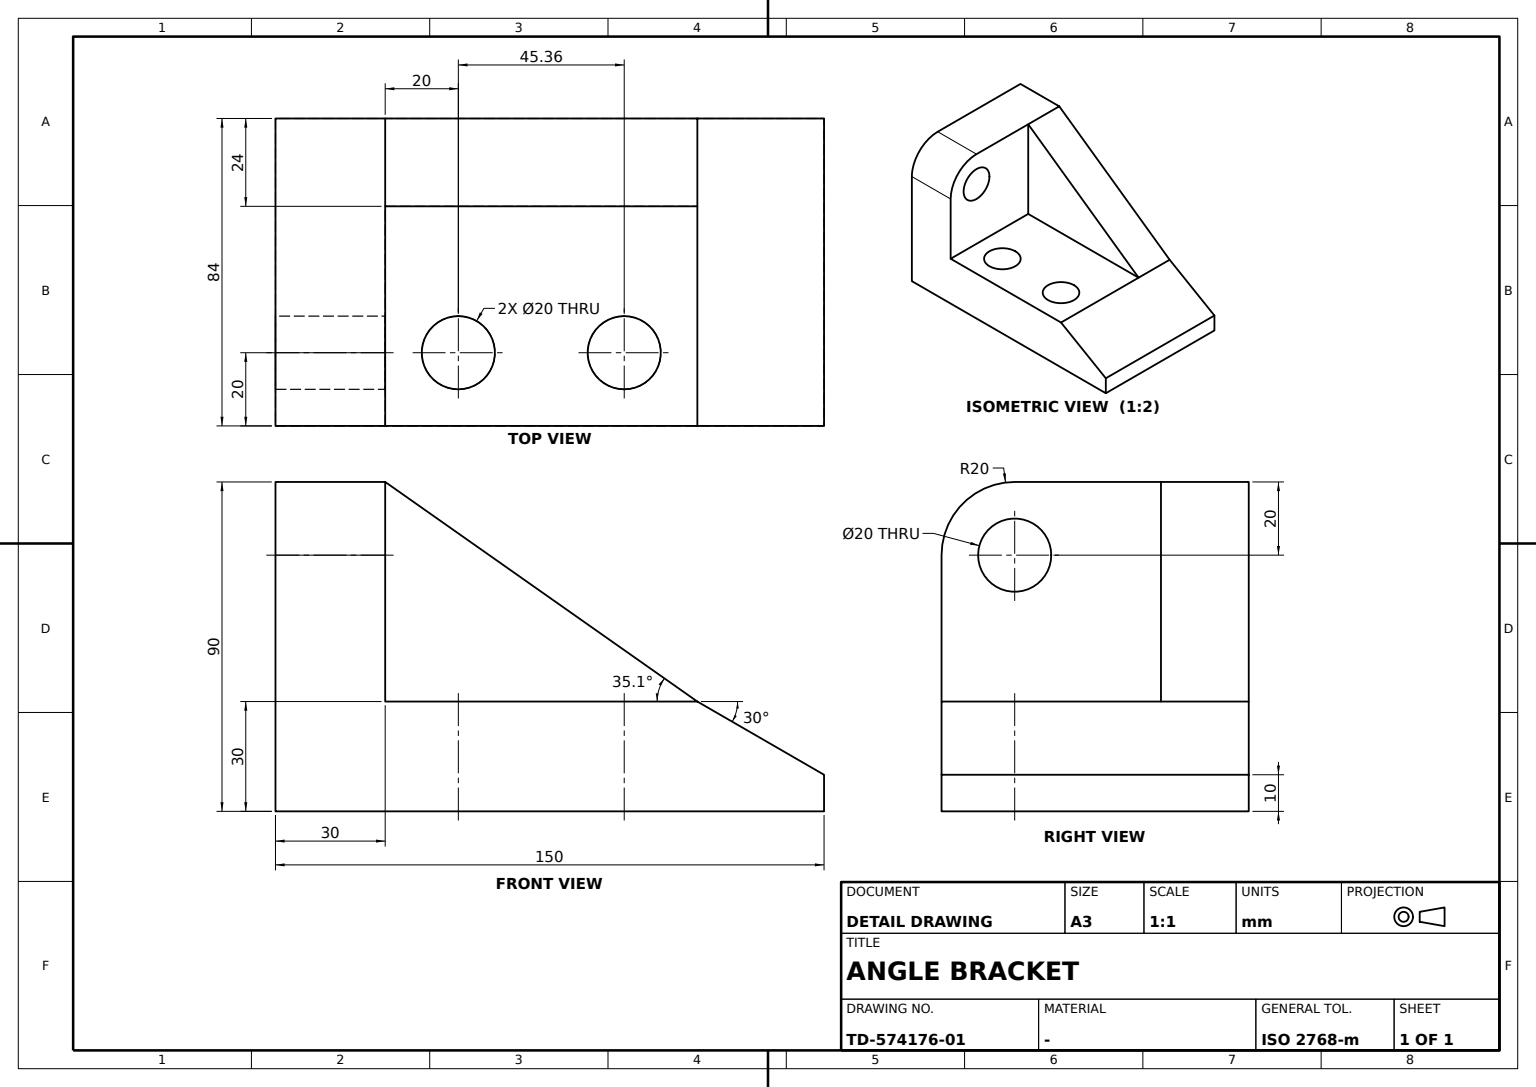
ISO-10303-21;
HEADER;
FILE_DESCRIPTION((''),'2;1');
FILE_NAME('','',(''),(''),'','','');
FILE_SCHEMA(('AUTOMOTIVE_DESIGN'));
ENDSEC;
DATA;
#1=APPLICATION_CONTEXT('');
#2=PRODUCT_CONTEXT('',#1,'mechanical');
#3=PRODUCT('','','',(#2));
#4=PRODUCT_DEFINITION_FORMATION('','',#3);
#5=PRODUCT_DEFINITION_CONTEXT('',#1,'design');
#6=PRODUCT_DEFINITION('','',#4,#5);
#7=PRODUCT_DEFINITION_SHAPE('','',#6);
#8=(LENGTH_UNIT()NAMED_UNIT(*)SI_UNIT(.MILLI.,.METRE.));
#9=(NAMED_UNIT(*)PLANE_ANGLE_UNIT()SI_UNIT($,.RADIAN.));
#10=(NAMED_UNIT(*)SI_UNIT($,.STERADIAN.)SOLID_ANGLE_UNIT());
#11=UNCERTAINTY_MEASURE_WITH_UNIT(LENGTH_MEASURE(1.E-05),#8,'distance_accuracy_value','');
#12=(GEOMETRIC_REPRESENTATION_CONTEXT(3)GLOBAL_UNCERTAINTY_ASSIGNED_CONTEXT((#11))GLOBAL_UNIT_ASSIGNED_CONTEXT((#8,#9,#10))REPRESENTATION_CONTEXT('',''));
#13=CARTESIAN_POINT('',(42.,150.,10.));
#14=VERTEX_POINT('',#13);
#15=CARTESIAN_POINT('',(-42.,150.,10.));
#16=VERTEX_POINT('',#15);
#17=CARTESIAN_POINT('',(0.,150.,10.));
#18=DIRECTION('',(-1.,0.,0.));
#19=VECTOR('',#18,1000.);
#20=LINE('',#17,#19);
#21=EDGE_CURVE('',#14,#16,#20,.T.);
#22=ORIENTED_EDGE('',*,*,#21,.F.);
#23=CARTESIAN_POINT('',(42.,150.,0.));
#24=VERTEX_POINT('',#23);
#25=CARTESIAN_POINT('',(42.,150.,5.));
#26=DIRECTION('',(0.,0.,1.));
#27=VECTOR('',#26,1000.);
#28=LINE('',#25,#27);
#29=EDGE_CURVE('',#24,#14,#28,.T.);
#30=ORIENTED_EDGE('',*,*,#29,.F.);
#31=CARTESIAN_POINT('',(-42.,150.,0.));
#32=VERTEX_POINT('',#31);
#33=CARTESIAN_POINT('',(0.,150.,0.));
#34=DIRECTION('',(1.,0.,0.));
#35=VECTOR('',#34,1000.);
#36=LINE('',#33,#35);
#37=EDGE_CURVE('',#32,#24,#36,.T.);
#38=ORIENTED_EDGE('',*,*,#37,.F.);
#39=CARTESIAN_POINT('',(-42.,150.,5.));
#40=LINE('',#39,#27);
#41=EDGE_CURVE('',#32,#16,#40,.T.);
#42=ORIENTED_EDGE('',*,*,#41,.T.);
#43=EDGE_LOOP('',(#22,#30,#38,#42));
#44=FACE_OUTER_BOUND('',#43,.T.);
#45=DIRECTION('',(0.,1.,0.));
#46=AXIS2_PLACEMENT_3D('',#33,#45,#26);
#47=PLANE('',#46);
#48=ADVANCED_FACE('',(#44),#47,.T.);
#49=CARTESIAN_POINT('',(-18.,30.,30.));
#50=VERTEX_POINT('',#49);
#51=CARTESIAN_POINT('',(42.,30.,30.));
#52=VERTEX_POINT('',#51);
#53=CARTESIAN_POINT('',(12.,30.,30.));
#54=LINE('',#53,#35);
#55=EDGE_CURVE('',#50,#52,#54,.T.);
#56=ORIENTED_EDGE('',*,*,#55,.F.);
#57=CARTESIAN_POINT('',(-18.,30.,90.));
#58=VERTEX_POINT('',#57);
#59=CARTESIAN_POINT('',(-18.,30.,60.));
#60=DIRECTION('',(0.,0.,-1.));
#61=VECTOR('',#60,1000.);
#62=LINE('',#59,#61);
#63=EDGE_CURVE('',#58,#50,#62,.T.);
#64=ORIENTED_EDGE('',*,*,#63,.F.);
#65=CARTESIAN_POINT('',(22.,30.,90.));
#66=VERTEX_POINT('',#65);
#67=CARTESIAN_POINT('',(2.,30.,90.));
#68=LINE('',#67,#35);
#69=EDGE_CURVE('',#58,#66,#68,.T.);
#70=ORIENTED_EDGE('',*,*,#69,.T.);
#71=CARTESIAN_POINT('',(42.,30.,70.));
#72=VERTEX_POINT('',#71);
#73=CARTESIAN_POINT('',(22.,30.,70.));
#74=DIRECTION('',(0.,-1.,0.));
#75=AXIS2_PLACEMENT_3D('',#73,#74,#60);
#76=CIRCLE('',#75,20.);
#77=EDGE_CURVE('',#72,#66,#76,.T.);
#78=ORIENTED_EDGE('',*,*,#77,.F.);
#79=CARTESIAN_POINT('',(42.,30.,50.));
#80=LINE('',#79,#27);
#81=EDGE_CURVE('',#52,#72,#80,.T.);
#82=ORIENTED_EDGE('',*,*,#81,.F.);
#83=EDGE_LOOP('',(#56,#64,#70,#78,#82));
#84=FACE_OUTER_BOUND('',#83,.T.);
#85=CARTESIAN_POINT('',(12.,30.,70.));
#86=VERTEX_POINT('',#85);
#87=CARTESIAN_POINT('',(32.,30.,70.));
#88=VERTEX_POINT('',#87);
#89=AXIS2_PLACEMENT_3D('',#73,#45,#18);
#90=CIRCLE('',#89,10.);
#91=EDGE_CURVE('',#86,#88,#90,.T.);
#92=ORIENTED_EDGE('',*,*,#91,.F.);
#93=EDGE_CURVE('',#88,#86,#90,.T.);
#94=ORIENTED_EDGE('',*,*,#93,.F.);
#95=EDGE_LOOP('',(#92,#94));
#96=FACE_BOUND('',#95,.T.);
#97=CARTESIAN_POINT('',(0.,30.,90.));
#98=AXIS2_PLACEMENT_3D('',#97,#74,#60);
#99=PLANE('',#98);
#100=ADVANCED_FACE('',(#84,#96),#99,.F.);
#101=ORIENTED_EDGE('',*,*,#41,.F.);
#102=CARTESIAN_POINT('',(-42.,0.,0.));
#103=VERTEX_POINT('',#102);
#104=CARTESIAN_POINT('',(-42.,75.,0.));
#105=VECTOR('',#45,1000.);
#106=LINE('',#104,#105);
#107=EDGE_CURVE('',#103,#32,#106,.T.);
#108=ORIENTED_EDGE('',*,*,#107,.F.);
#109=CARTESIAN_POINT('',(-42.,0.,90.));
#110=VERTEX_POINT('',#109);
#111=CARTESIAN_POINT('',(-42.,0.,45.));
#112=LINE('',#111,#61);
#113=EDGE_CURVE('',#110,#103,#112,.T.);
#114=ORIENTED_EDGE('',*,*,#113,.F.);
#115=CARTESIAN_POINT('',(-42.,30.,90.));
#116=VERTEX_POINT('',#115);
#117=CARTESIAN_POINT('',(-42.,15.,90.));
#118=VECTOR('',#74,1000.);
#119=LINE('',#117,#118);
#120=EDGE_CURVE('',#116,#110,#119,.T.);
#121=ORIENTED_EDGE('',*,*,#120,.F.);
#122=CARTESIAN_POINT('',(-42.,115.358984,30.));
#123=VERTEX_POINT('',#122);
#124=CARTESIAN_POINT('',(-42.,72.679492,60.));
#125=DIRECTION('',(0.,-0.818110482,0.575061074));
#126=VECTOR('',#125,1000.);
#127=LINE('',#124,#126);
#128=EDGE_CURVE('',#123,#116,#127,.T.);
#129=ORIENTED_EDGE('',*,*,#128,.F.);
#130=CARTESIAN_POINT('',(-42.,132.679492,20.));
#131=DIRECTION('',(0.,-0.866025404,0.5));
#132=VECTOR('',#131,1000.);
#133=LINE('',#130,#132);
#134=EDGE_CURVE('',#16,#123,#133,.T.);
#135=ORIENTED_EDGE('',*,*,#134,.F.);
#136=EDGE_LOOP('',(#101,#108,#114,#121,#129,#135));
#137=FACE_OUTER_BOUND('',#136,.T.);
#138=AXIS2_PLACEMENT_3D('',#102,#34,#45);
#139=PLANE('',#138);
#140=ADVANCED_FACE('',(#137),#139,.F.);
#141=CARTESIAN_POINT('',(12.,0.,70.));
#142=VERTEX_POINT('',#141);
#143=CARTESIAN_POINT('',(32.,0.,70.));
#144=VERTEX_POINT('',#143);
#145=CARTESIAN_POINT('',(22.,0.,70.));
#146=AXIS2_PLACEMENT_3D('',#145,#45,#26);
#147=CIRCLE('',#146,10.);
#148=EDGE_CURVE('',#142,#144,#147,.T.);
#149=ORIENTED_EDGE('',*,*,#148,.T.);
#150=EDGE_CURVE('',#144,#142,#147,.T.);
#151=ORIENTED_EDGE('',*,*,#150,.T.);
#152=EDGE_LOOP('',(#149,#151));
#153=FACE_BOUND('',#152,.T.);
#154=ORIENTED_EDGE('',*,*,#113,.T.);
#155=CARTESIAN_POINT('',(42.,0.,0.));
#156=VERTEX_POINT('',#155);
#157=CARTESIAN_POINT('',(0.,0.,0.));
#158=LINE('',#157,#35);
#159=EDGE_CURVE('',#103,#156,#158,.T.);
#160=ORIENTED_EDGE('',*,*,#159,.T.);
#161=CARTESIAN_POINT('',(42.,0.,70.));
#162=VERTEX_POINT('',#161);
#163=CARTESIAN_POINT('',(42.,0.,35.));
#164=LINE('',#163,#61);
#165=EDGE_CURVE('',#162,#156,#164,.T.);
#166=ORIENTED_EDGE('',*,*,#165,.F.);
#167=CARTESIAN_POINT('',(22.,0.,90.));
#168=VERTEX_POINT('',#167);
#169=CIRCLE('',#146,20.);
#170=EDGE_CURVE('',#168,#162,#169,.T.);
#171=ORIENTED_EDGE('',*,*,#170,.F.);
#172=CARTESIAN_POINT('',(-10.,0.,90.));
#173=LINE('',#172,#35);
#174=EDGE_CURVE('',#110,#168,#173,.T.);
#175=ORIENTED_EDGE('',*,*,#174,.F.);
#176=EDGE_LOOP('',(#154,#160,#166,#171,#175));
#177=FACE_OUTER_BOUND('',#176,.T.);
#178=AXIS2_PLACEMENT_3D('',#157,#45,#26);
#179=PLANE('',#178);
#180=ADVANCED_FACE('',(#153,#177),#179,.F.);
#181=CARTESIAN_POINT('',(12.,95.358984,0.));
#182=VERTEX_POINT('',#181);
#183=CARTESIAN_POINT('',(32.,95.358984,0.));
#184=VERTEX_POINT('',#183);
#185=CARTESIAN_POINT('',(22.,95.358984,0.));
#186=AXIS2_PLACEMENT_3D('',#185,#60,#34);
#187=CIRCLE('',#186,10.);
#188=EDGE_CURVE('',#182,#184,#187,.T.);
#189=ORIENTED_EDGE('',*,*,#188,.T.);
#190=CARTESIAN_POINT('',(32.,95.358984,30.));
#191=VERTEX_POINT('',#190);
#192=CARTESIAN_POINT('',(32.,95.358984,45.155));
#193=LINE('',#192,#27);
#194=EDGE_CURVE('',#184,#191,#193,.T.);
#195=ORIENTED_EDGE('',*,*,#194,.T.);
#196=CARTESIAN_POINT('',(12.,95.358984,30.));
#197=VERTEX_POINT('',#196);
#198=CARTESIAN_POINT('',(22.,95.358984,30.));
#199=AXIS2_PLACEMENT_3D('',#198,#60,#45);
#200=CIRCLE('',#199,10.);
#201=EDGE_CURVE('',#197,#191,#200,.T.);
#202=ORIENTED_EDGE('',*,*,#201,.F.);
#203=CARTESIAN_POINT('',(12.,95.358984,45.155));
#204=LINE('',#203,#27);
#205=EDGE_CURVE('',#182,#197,#204,.T.);
#206=ORIENTED_EDGE('',*,*,#205,.F.);
#207=EDGE_LOOP('',(#189,#195,#202,#206));
#208=FACE_OUTER_BOUND('',#207,.T.);
#209=AXIS2_PLACEMENT_3D('',#198,#26,#34);
#210=CYLINDRICAL_SURFACE('',#209,10.);
#211=ADVANCED_FACE('',(#208),#210,.F.);
#212=ORIENTED_EDGE('',*,*,#194,.F.);
#213=EDGE_CURVE('',#184,#182,#187,.T.);
#214=ORIENTED_EDGE('',*,*,#213,.T.);
#215=ORIENTED_EDGE('',*,*,#205,.T.);
#216=EDGE_CURVE('',#191,#197,#200,.T.);
#217=ORIENTED_EDGE('',*,*,#216,.F.);
#218=EDGE_LOOP('',(#212,#214,#215,#217));
#219=FACE_OUTER_BOUND('',#218,.T.);
#220=ADVANCED_FACE('',(#219),#210,.F.);
#221=ORIENTED_EDGE('',*,*,#128,.T.);
#222=CARTESIAN_POINT('',(-30.,30.,90.));
#223=LINE('',#222,#35);
#224=EDGE_CURVE('',#116,#58,#223,.T.);
#225=ORIENTED_EDGE('',*,*,#224,.T.);
#226=CARTESIAN_POINT('',(-18.,115.358984,30.));
#227=VERTEX_POINT('',#226);
#228=CARTESIAN_POINT('',(-18.,72.679492,60.));
#229=LINE('',#228,#126);
#230=EDGE_CURVE('',#227,#58,#229,.T.);
#231=ORIENTED_EDGE('',*,*,#230,.F.);
#232=CARTESIAN_POINT('',(-30.,115.358984,30.));
#233=LINE('',#232,#19);
#234=EDGE_CURVE('',#227,#123,#233,.T.);
#235=ORIENTED_EDGE('',*,*,#234,.T.);
#236=EDGE_LOOP('',(#221,#225,#231,#235));
#237=FACE_OUTER_BOUND('',#236,.T.);
#238=DIRECTION('',(0.,-0.575061074,-0.818110482));
#239=DIRECTION('',(0.,0.818110482,-0.575061074));
#240=AXIS2_PLACEMENT_3D('',#122,#238,#239);
#241=PLANE('',#240);
#242=ADVANCED_FACE('',(#237),#241,.F.);
#243=ORIENTED_EDGE('',*,*,#29,.T.);
#244=CARTESIAN_POINT('',(42.,115.358984,30.));
#245=VERTEX_POINT('',#244);
#246=CARTESIAN_POINT('',(42.,132.679492,20.));
#247=DIRECTION('',(0.,0.866025404,-0.5));
#248=VECTOR('',#247,1000.);
#249=LINE('',#246,#248);
#250=EDGE_CURVE('',#245,#14,#249,.T.);
#251=ORIENTED_EDGE('',*,*,#250,.F.);
#252=CARTESIAN_POINT('',(42.,72.679492,30.));
#253=LINE('',#252,#118);
#254=EDGE_CURVE('',#245,#52,#253,.T.);
#255=ORIENTED_EDGE('',*,*,#254,.T.);
#256=ORIENTED_EDGE('',*,*,#81,.T.);
#257=CARTESIAN_POINT('',(42.,15.,70.));
#258=LINE('',#257,#118);
#259=EDGE_CURVE('',#72,#162,#258,.T.);
#260=ORIENTED_EDGE('',*,*,#259,.T.);
#261=ORIENTED_EDGE('',*,*,#165,.T.);
#262=CARTESIAN_POINT('',(42.,75.,0.));
#263=LINE('',#262,#105);
#264=EDGE_CURVE('',#156,#24,#263,.T.);
#265=ORIENTED_EDGE('',*,*,#264,.T.);
#266=EDGE_LOOP('',(#243,#251,#255,#256,#260,#261,#265));
#267=FACE_OUTER_BOUND('',#266,.T.);
#268=AXIS2_PLACEMENT_3D('',#155,#34,#45);
#269=PLANE('',#268);
#270=ADVANCED_FACE('',(#267),#269,.T.);
#271=CARTESIAN_POINT('',(32.,14.34,70.));
#272=LINE('',#271,#118);
#273=EDGE_CURVE('',#88,#144,#272,.T.);
#274=ORIENTED_EDGE('',*,*,#273,.F.);
#275=ORIENTED_EDGE('',*,*,#93,.T.);
#276=CARTESIAN_POINT('',(12.,14.34,70.));
#277=LINE('',#276,#118);
#278=EDGE_CURVE('',#86,#142,#277,.T.);
#279=ORIENTED_EDGE('',*,*,#278,.T.);
#280=ORIENTED_EDGE('',*,*,#150,.F.);
#281=EDGE_LOOP('',(#274,#275,#279,#280));
#282=FACE_OUTER_BOUND('',#281,.T.);
#283=CARTESIAN_POINT('',(22.,14.34,70.));
#284=AXIS2_PLACEMENT_3D('',#283,#74,#18);
#285=CYLINDRICAL_SURFACE('',#284,10.);
#286=ADVANCED_FACE('',(#282),#285,.F.);
#287=ORIENTED_EDGE('',*,*,#134,.T.);
#288=ORIENTED_EDGE('',*,*,#234,.F.);
#289=CARTESIAN_POINT('',(12.,115.358984,30.));
#290=LINE('',#289,#19);
#291=EDGE_CURVE('',#245,#227,#290,.T.);
#292=ORIENTED_EDGE('',*,*,#291,.F.);
#293=ORIENTED_EDGE('',*,*,#250,.T.);
#294=ORIENTED_EDGE('',*,*,#21,.T.);
#295=EDGE_LOOP('',(#287,#288,#292,#293,#294));
#296=FACE_OUTER_BOUND('',#295,.T.);
#297=DIRECTION('',(0.,-0.5,-0.866025404));
#298=AXIS2_PLACEMENT_3D('',#13,#297,#131);
#299=PLANE('',#298);
#300=ADVANCED_FACE('',(#296),#299,.F.);
#301=ORIENTED_EDGE('',*,*,#224,.F.);
#302=ORIENTED_EDGE('',*,*,#120,.T.);
#303=ORIENTED_EDGE('',*,*,#174,.T.);
#304=CARTESIAN_POINT('',(22.,15.,90.));
#305=LINE('',#304,#118);
#306=EDGE_CURVE('',#66,#168,#305,.T.);
#307=ORIENTED_EDGE('',*,*,#306,.F.);
#308=ORIENTED_EDGE('',*,*,#69,.F.);
#309=EDGE_LOOP('',(#301,#302,#303,#307,#308));
#310=FACE_OUTER_BOUND('',#309,.T.);
#311=CARTESIAN_POINT('',(0.,0.,90.));
#312=AXIS2_PLACEMENT_3D('',#311,#60,#45);
#313=PLANE('',#312);
#314=ADVANCED_FACE('',(#310),#313,.F.);
#315=CARTESIAN_POINT('',(-18.,72.679492,30.));
#316=LINE('',#315,#105);
#317=EDGE_CURVE('',#50,#227,#316,.T.);
#318=ORIENTED_EDGE('',*,*,#317,.T.);
#319=ORIENTED_EDGE('',*,*,#230,.T.);
#320=ORIENTED_EDGE('',*,*,#63,.T.);
#321=EDGE_LOOP('',(#318,#319,#320));
#322=FACE_OUTER_BOUND('',#321,.T.);
#323=CARTESIAN_POINT('',(-18.,0.,0.));
#324=AXIS2_PLACEMENT_3D('',#323,#18,#74);
#325=PLANE('',#324);
#326=ADVANCED_FACE('',(#322),#325,.F.);
#327=ORIENTED_EDGE('',*,*,#77,.T.);
#328=ORIENTED_EDGE('',*,*,#306,.T.);
#329=ORIENTED_EDGE('',*,*,#170,.T.);
#330=ORIENTED_EDGE('',*,*,#259,.F.);
#331=EDGE_LOOP('',(#327,#328,#329,#330));
#332=FACE_OUTER_BOUND('',#331,.T.);
#333=CARTESIAN_POINT('',(22.,75.,70.));
#334=AXIS2_PLACEMENT_3D('',#333,#74,#26);
#335=CYLINDRICAL_SURFACE('',#334,20.);
#336=ADVANCED_FACE('',(#332),#335,.T.);
#337=CARTESIAN_POINT('',(32.,50.,30.));
#338=VERTEX_POINT('',#337);
#339=CARTESIAN_POINT('',(32.,50.,0.));
#340=VERTEX_POINT('',#339);
#341=CARTESIAN_POINT('',(32.,50.,14.34));
#342=LINE('',#341,#61);
#343=EDGE_CURVE('',#338,#340,#342,.T.);
#344=ORIENTED_EDGE('',*,*,#343,.T.);
#345=CARTESIAN_POINT('',(12.,50.,0.));
#346=VERTEX_POINT('',#345);
#347=CARTESIAN_POINT('',(22.,50.,0.));
#348=AXIS2_PLACEMENT_3D('',#347,#60,#45);
#349=CIRCLE('',#348,10.);
#350=EDGE_CURVE('',#340,#346,#349,.T.);
#351=ORIENTED_EDGE('',*,*,#350,.T.);
#352=CARTESIAN_POINT('',(12.,50.,30.));
#353=VERTEX_POINT('',#352);
#354=CARTESIAN_POINT('',(12.,50.,14.34));
#355=LINE('',#354,#61);
#356=EDGE_CURVE('',#353,#346,#355,.T.);
#357=ORIENTED_EDGE('',*,*,#356,.F.);
#358=CARTESIAN_POINT('',(22.,50.,30.));
#359=AXIS2_PLACEMENT_3D('',#358,#26,#34);
#360=CIRCLE('',#359,10.);
#361=EDGE_CURVE('',#353,#338,#360,.T.);
#362=ORIENTED_EDGE('',*,*,#361,.T.);
#363=EDGE_LOOP('',(#344,#351,#357,#362));
#364=FACE_OUTER_BOUND('',#363,.T.);
#365=CARTESIAN_POINT('',(22.,50.,14.34));
#366=AXIS2_PLACEMENT_3D('',#365,#60,#34);
#367=CYLINDRICAL_SURFACE('',#366,10.);
#368=ADVANCED_FACE('',(#364),#367,.F.);
#369=ORIENTED_EDGE('',*,*,#188,.F.);
#370=ORIENTED_EDGE('',*,*,#213,.F.);
#371=EDGE_LOOP('',(#369,#370));
#372=FACE_BOUND('',#371,.T.);
#373=EDGE_CURVE('',#346,#340,#349,.T.);
#374=ORIENTED_EDGE('',*,*,#373,.F.);
#375=ORIENTED_EDGE('',*,*,#350,.F.);
#376=EDGE_LOOP('',(#374,#375));
#377=FACE_BOUND('',#376,.T.);
#378=ORIENTED_EDGE('',*,*,#37,.T.);
#379=ORIENTED_EDGE('',*,*,#264,.F.);
#380=ORIENTED_EDGE('',*,*,#159,.F.);
#381=ORIENTED_EDGE('',*,*,#107,.T.);
#382=EDGE_LOOP('',(#378,#379,#380,#381));
#383=FACE_OUTER_BOUND('',#382,.T.);
#384=AXIS2_PLACEMENT_3D('',#157,#60,#45);
#385=PLANE('',#384);
#386=ADVANCED_FACE('',(#372,#377,#383),#385,.T.);
#387=ORIENTED_EDGE('',*,*,#273,.T.);
#388=ORIENTED_EDGE('',*,*,#148,.F.);
#389=ORIENTED_EDGE('',*,*,#278,.F.);
#390=ORIENTED_EDGE('',*,*,#91,.T.);
#391=EDGE_LOOP('',(#387,#388,#389,#390));
#392=FACE_OUTER_BOUND('',#391,.T.);
#393=ADVANCED_FACE('',(#392),#285,.F.);
#394=ORIENTED_EDGE('',*,*,#373,.T.);
#395=ORIENTED_EDGE('',*,*,#343,.F.);
#396=EDGE_CURVE('',#338,#353,#360,.T.);
#397=ORIENTED_EDGE('',*,*,#396,.T.);
#398=ORIENTED_EDGE('',*,*,#356,.T.);
#399=EDGE_LOOP('',(#394,#395,#397,#398));
#400=FACE_OUTER_BOUND('',#399,.T.);
#401=ADVANCED_FACE('',(#400),#367,.F.);
#402=ORIENTED_EDGE('',*,*,#201,.T.);
#403=ORIENTED_EDGE('',*,*,#216,.T.);
#404=EDGE_LOOP('',(#402,#403));
#405=FACE_BOUND('',#404,.T.);
#406=ORIENTED_EDGE('',*,*,#361,.F.);
#407=ORIENTED_EDGE('',*,*,#396,.F.);
#408=EDGE_LOOP('',(#406,#407));
#409=FACE_BOUND('',#408,.T.);
#410=ORIENTED_EDGE('',*,*,#254,.F.);
#411=ORIENTED_EDGE('',*,*,#291,.T.);
#412=ORIENTED_EDGE('',*,*,#317,.F.);
#413=ORIENTED_EDGE('',*,*,#55,.T.);
#414=EDGE_LOOP('',(#410,#411,#412,#413));
#415=FACE_OUTER_BOUND('',#414,.T.);
#416=CARTESIAN_POINT('',(0.,30.,30.));
#417=AXIS2_PLACEMENT_3D('',#416,#60,#45);
#418=PLANE('',#417);
#419=ADVANCED_FACE('',(#405,#409,#415),#418,.F.);
#420=CLOSED_SHELL('',(#48,#100,#140,#180,#211,#220,#242,#270,#286,#300,#314,#326,#336,#368,#386,#393,#401,#419));
#421=MANIFOLD_SOLID_BREP('',#420);
#422=ADVANCED_BREP_SHAPE_REPRESENTATION('',(#421),#12);
#423=SHAPE_DEFINITION_REPRESENTATION(#7,#422);
ENDSEC;
END-ISO-10303-21;
